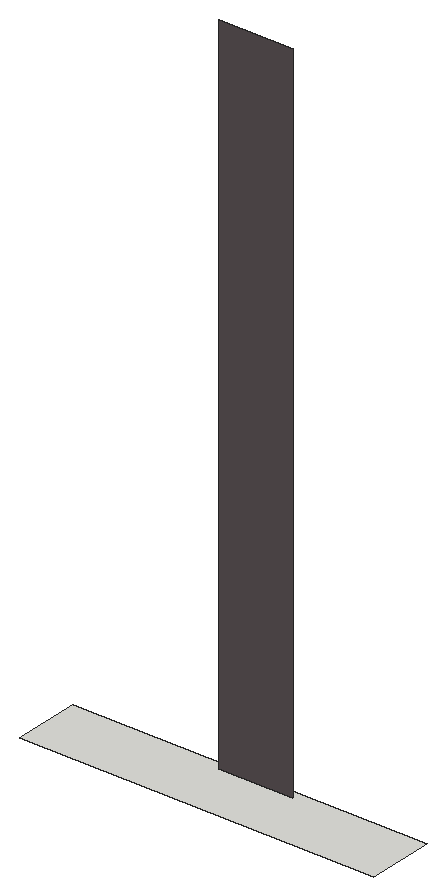
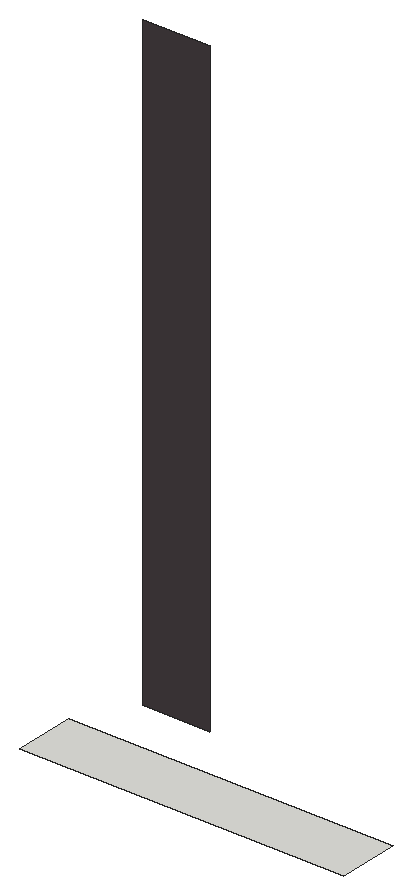
# SketchUp Ruby script. Lengths in inches.
U = 1.inch
M = Sketchup.active_model
def pt(a) = Geom::Point3d.new(a.map { |v| v * U })
def face(e, loops, mat)
  f = e.add_face(loops[0].map { |a| pt(a) })
  loops[1..].each { |l| e.add_face(l.map { |a| pt(a) }).erase! }
  f.material = f.back_material = mat if mat
  f
end
# faces: each face lists its corners as indices into pts; further lists are holes
def faces(e, pts, list, mat = nil) = list.each { |f| face(e, (f[0].is_a?(Array) ? f : [f]).map { |l| l.map { |i| pts[i] } }, mat) }
# xy, xz, yz: faces in a plane at the given z, y or x. An outline is a flat list of corners, or four numbers for a rectangle; further outlines are holes
def ring(l) = l.size == 4 ? [[l[0], l[1]], [l[2], l[1]], [l[2], l[3]], [l[0], l[3]]] : l.each_slice(2).to_a
def flat(e, list, mat, &to3) = list.each { |f| face(e, (f[0].is_a?(Array) ? f : [f]).map { |l| ring(l).map { |u, v| to3.(u, v) } }, mat) }
def xy(e, z, list, mat = nil) = flat(e, list, mat) { |x, y| [x, y, z] }
def xz(e, y, list, mat = nil) = flat(e, list, mat) { |x, z| [x, y, z] }
def yz(e, x, list, mat = nil) = flat(e, list, mat) { |y, z| [x, y, z] }
def lines(e, pts, list) = list.each { |a, b| e.add_line(pt(pts[a]), pt(pts[b])) }
# prism: a flat outline (further loops are holes) pulled along v
def prism(e, loops, v, mat = nil)
  f = face(e, loops, mat); d = Geom::Vector3d.new(v.map { |x| x * U })
  f.pushpull(f.normal.samedirection?(d) ? d.length : -d.length)
end
def box(e, o, s, mat = nil) = prism(e, [[o, [o[0] + s[0], o[1], o[2]], [o[0] + s[0], o[1] + s[1], o[2]], [o[0], o[1] + s[1], o[2]]]], [0, 0, s[2]], mat)
def at(x, y, z, deg = 0) = Geom::Transformation.translation(pt([x, y, z])) * Geom::Transformation.rotation(ORIGIN, Z_AXIS, deg.degrees)
def axes(o, x, y, z) = Geom::Transformation.new([*x, 0, *y, 0, *z, 0, *pt(o).to_a, 1])
def part(name) = M.definitions.add(name)
# library, detail: a bought-in or finely detailed component or shape, given as its bounding box
def library(name, o, s) = part(name).tap { |d| box(d.entities, o, s) }
def detail(e, o, s) = box(e.add_group.entities, o, s)
def put(e, d, t, mat = nil) = e.add_instance(d, t).tap { |i| i.material = mat if mat }
def group(e, t, mat = nil) = e.add_group.tap { |g| g.transformation = t; g.material = mat if mat }.entities
root = M.entities
M.materials.add("[Asphalt New]").color = [91, 82, 84]
xy(root,15.61,[[330.33,92.3,351.27,96.24]])
xz(root,92.3,[[342.12,18.11,346.48,57.8125]],"[Asphalt New]")
